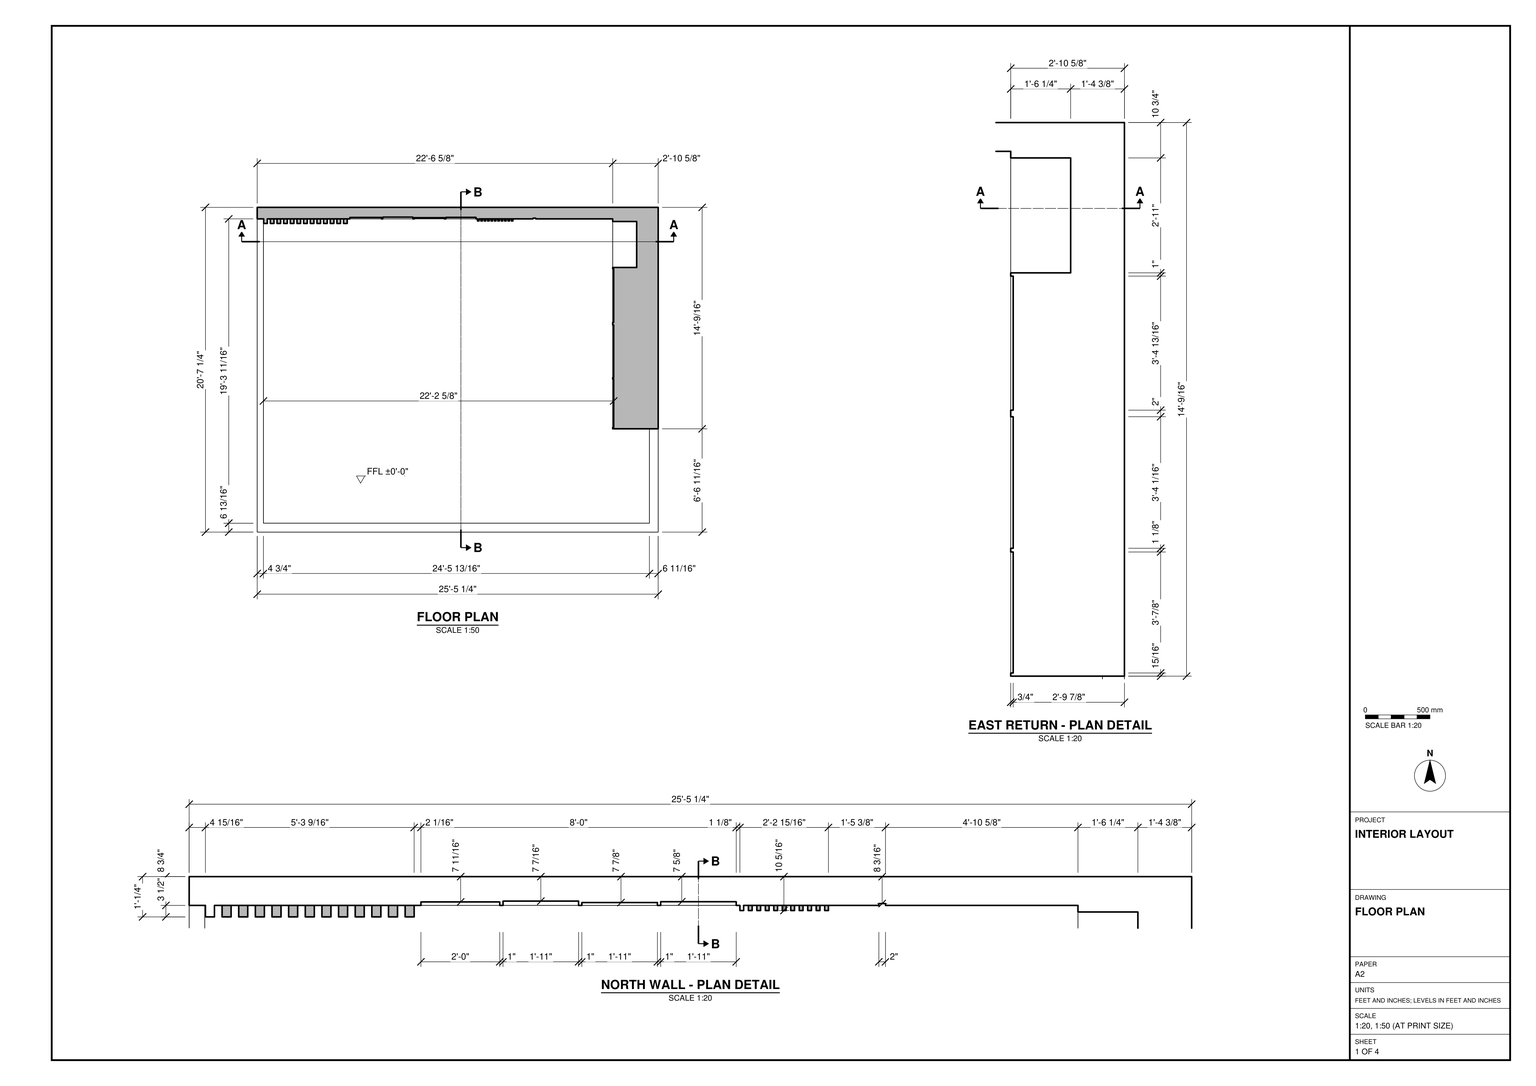
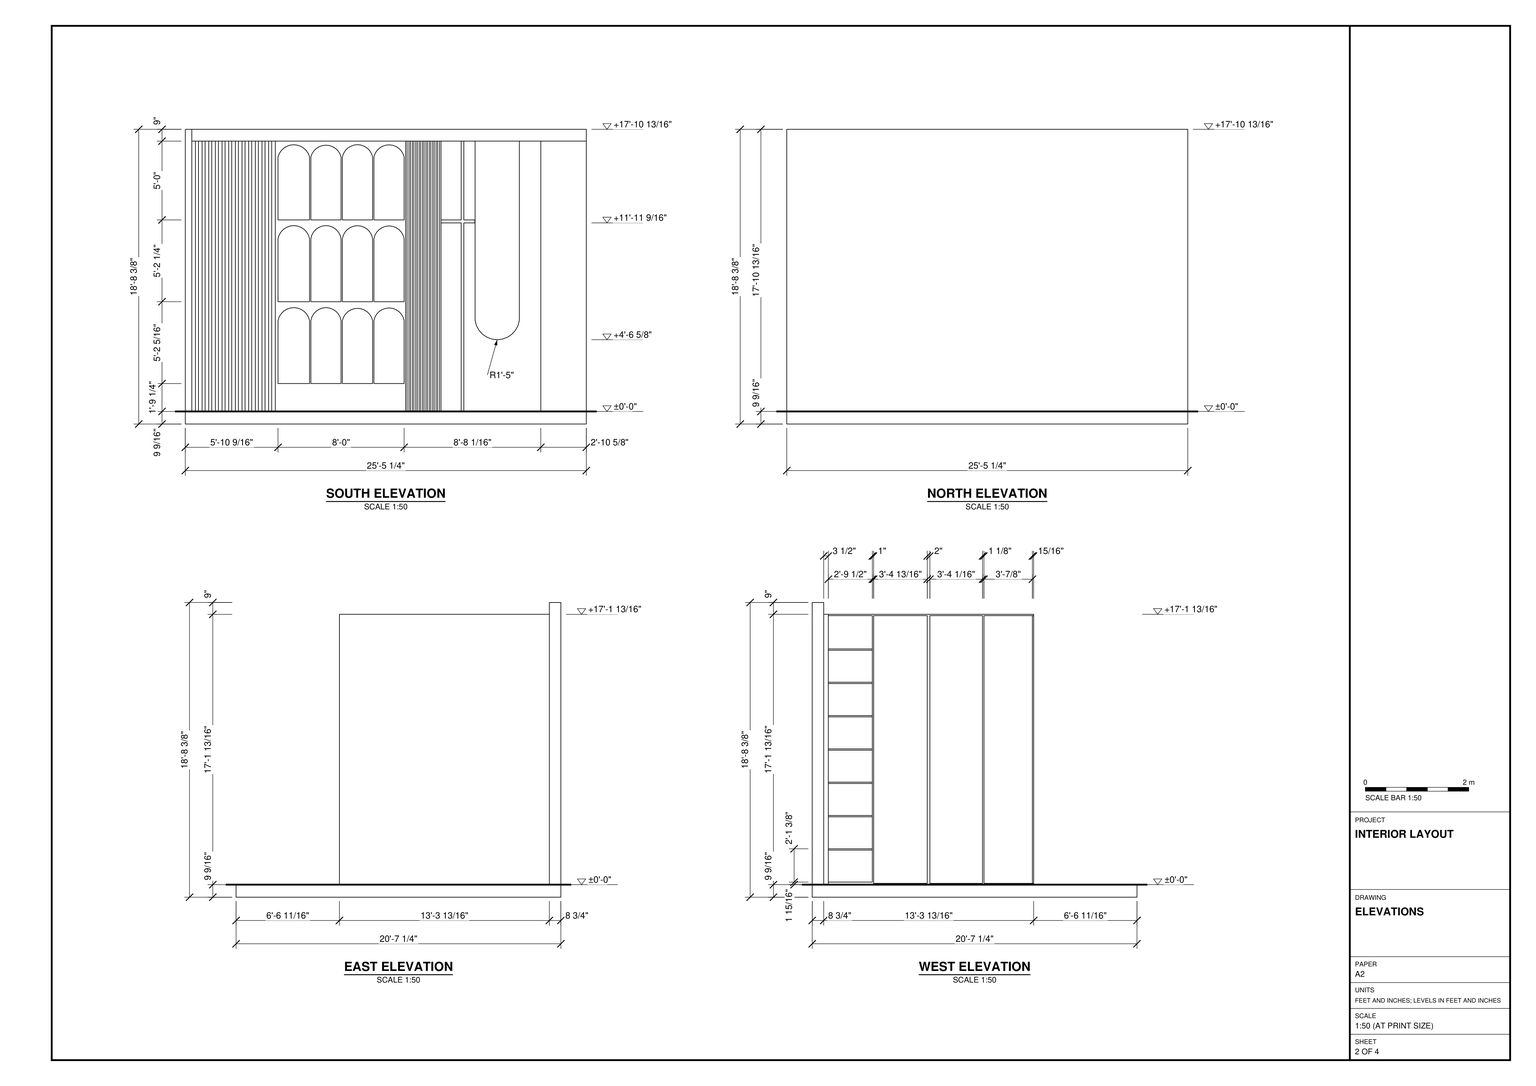
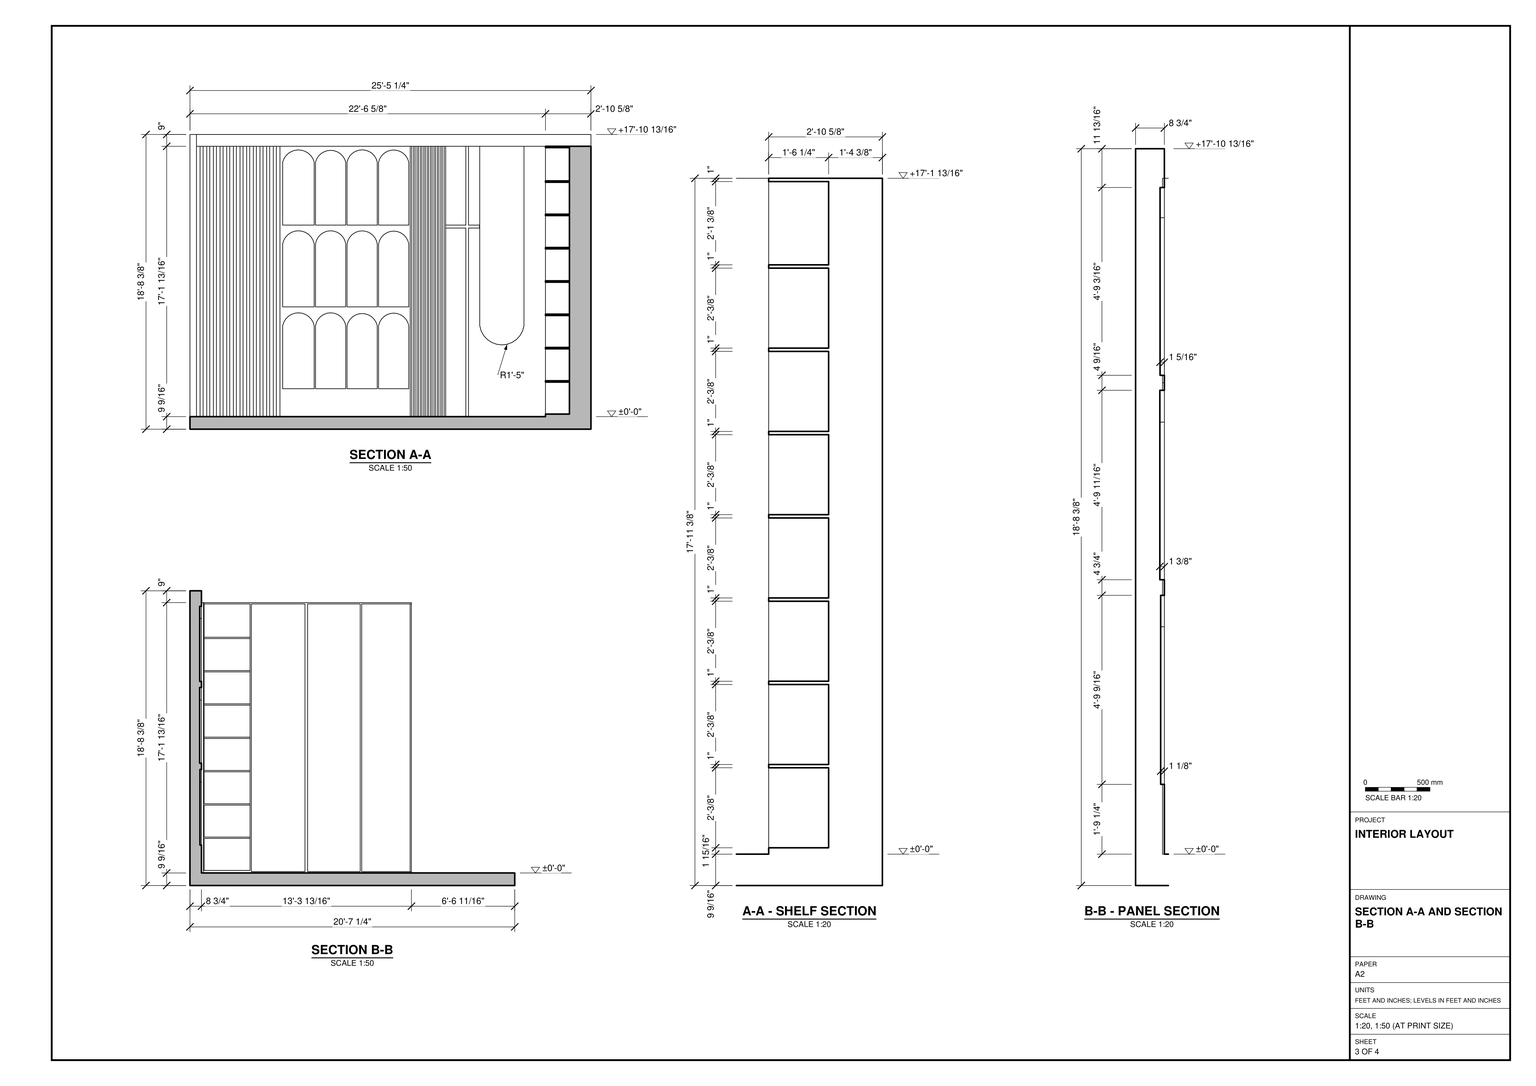
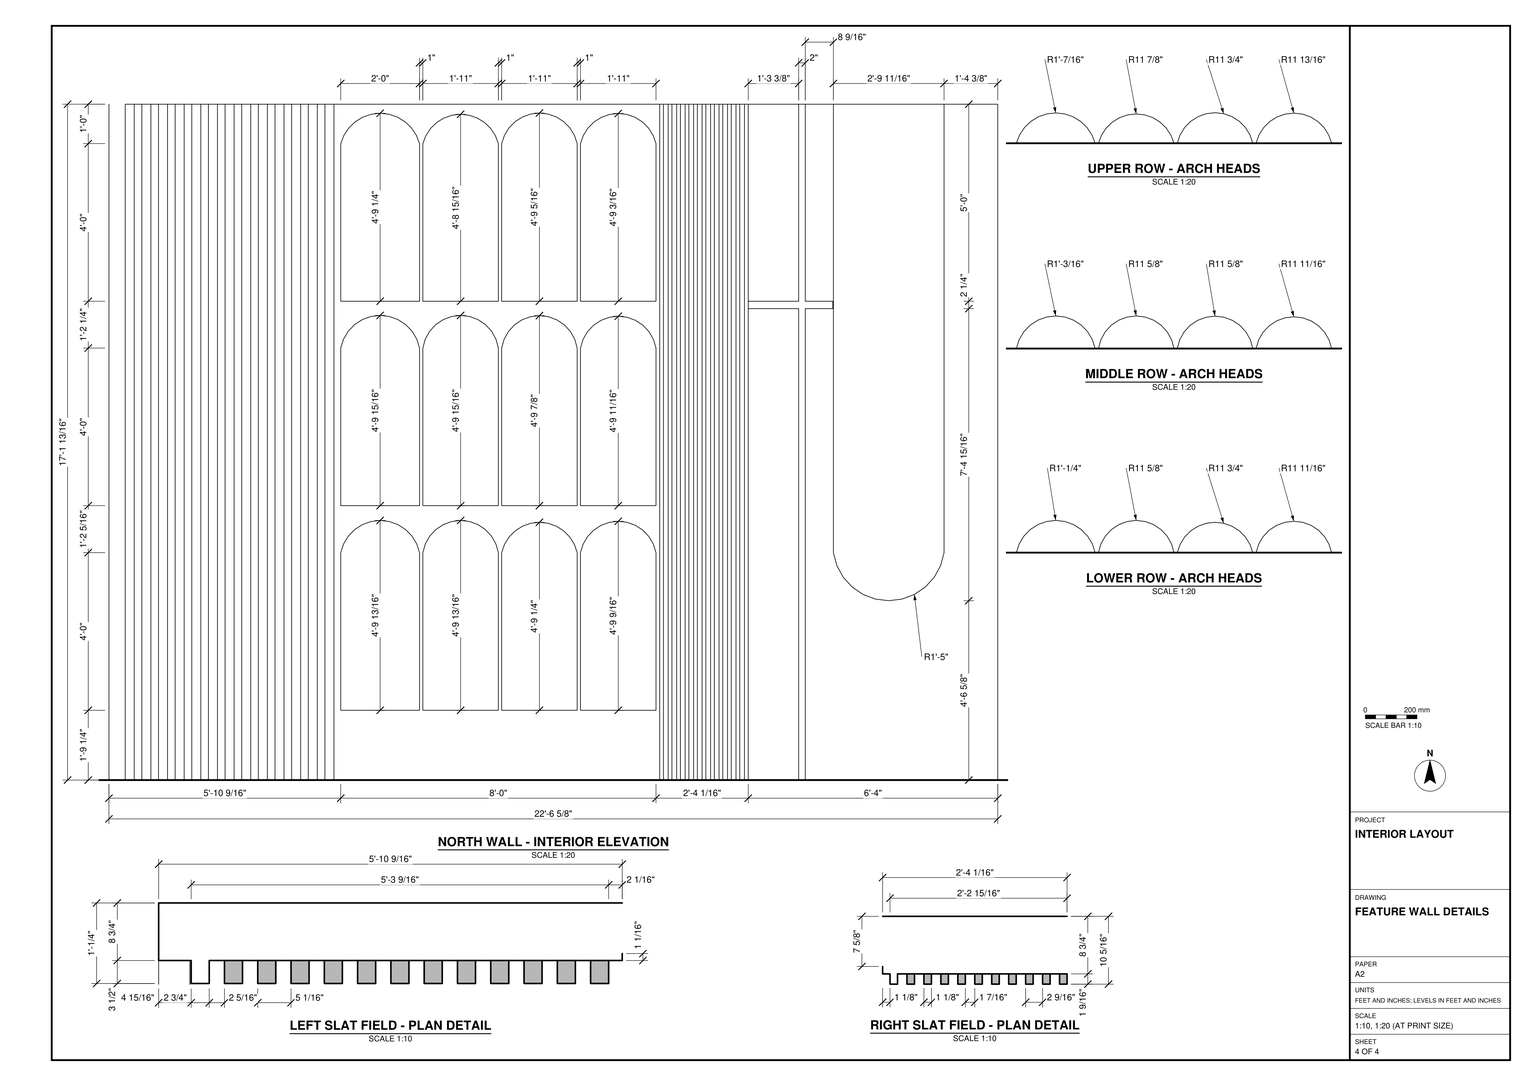
Use task_files/diagram_01.pdf to model the interior in SketchUp. Work in feet and inches. Set the finished floor at ±0'-0". The overall model measures 25'-5 1/4" east to west, 20'-7 1/4" north to south and 18'-8 3/8" from the underside of the slab to the top of the north wall.

Build the rectangular floor slab, the full-width north wall and the shorter east return. Use the plan details and sections for the wall thicknesses, panel offsets and shelf depths. On the room face of the north wall, place the field of round-headed panels between the broad and narrow bands of vertical slats. Follow the south elevation for the spacing of the arches, the clear strip above them and the tall panel with a rounded lower end toward the east corner. On the east return, place the open shelving nearest the north wall and the tall plain panels farther south. Leave the floor beyond the end of the return open as drawn.

Keep the slab, walls and individual joinery pieces in separate groups or components, and use components for repeated parts. Any decor or loose items shown may be represented by suitable library components. Save one SketchUp model as output_files/north_feature_wall_and_east_shelving_return.skp.

# SketchUp Ruby script. Lengths in inches.
U = 1.inch
M = Sketchup.active_model
def pt(a) = Geom::Point3d.new(a.map { |v| v * U })
def face(e, loops, mat)
  f = e.add_face(loops[0].map { |a| pt(a) })
  loops[1..].each { |l| e.add_face(l.map { |a| pt(a) }).erase! }
  f.material = f.back_material = mat if mat
  f
end
# faces: each face lists its corners as indices into pts; further lists are holes
def faces(e, pts, list, mat = nil) = list.each { |f| face(e, (f[0].is_a?(Array) ? f : [f]).map { |l| l.map { |i| pts[i] } }, mat) }
# xy, xz, yz: faces in a plane at the given z, y or x. An outline is a flat list of corners, or four numbers for a rectangle; further outlines are holes
def ring(l) = l.size == 4 ? [[l[0], l[1]], [l[2], l[1]], [l[2], l[3]], [l[0], l[3]]] : l.each_slice(2).to_a
def flat(e, list, mat, &to3) = list.each { |f| face(e, (f[0].is_a?(Array) ? f : [f]).map { |l| ring(l).map { |u, v| to3.(u, v) } }, mat) }
def xy(e, z, list, mat = nil) = flat(e, list, mat) { |x, y| [x, y, z] }
def xz(e, y, list, mat = nil) = flat(e, list, mat) { |x, z| [x, y, z] }
def yz(e, x, list, mat = nil) = flat(e, list, mat) { |y, z| [x, y, z] }
def lines(e, pts, list) = list.each { |a, b| e.add_line(pt(pts[a]), pt(pts[b])) }
# prism: a flat outline (further loops are holes) pulled along v
def prism(e, loops, v, mat = nil)
  f = face(e, loops, mat); d = Geom::Vector3d.new(v.map { |x| x * U })
  f.pushpull(f.normal.samedirection?(d) ? d.length : -d.length)
end
def box(e, o, s, mat = nil) = prism(e, [[o, [o[0] + s[0], o[1], o[2]], [o[0] + s[0], o[1] + s[1], o[2]], [o[0], o[1] + s[1], o[2]]]], [0, 0, s[2]], mat)
def at(x, y, z, deg = 0) = Geom::Transformation.translation(pt([x, y, z])) * Geom::Transformation.rotation(ORIGIN, Z_AXIS, deg.degrees)
def axes(o, x, y, z) = Geom::Transformation.new([*x, 0, *y, 0, *z, 0, *pt(o).to_a, 1])
def part(name) = M.definitions.add(name)
# library, detail: a bought-in or finely detailed component or shape, given as its bounding box
def library(name, o, s) = part(name).tap { |d| box(d.entities, o, s) }
def detail(e, o, s) = box(e.add_group.entities, o, s)
def put(e, d, t, mat = nil) = e.add_instance(d, t).tap { |i| i.material = mat if mat }
def group(e, t, mat = nil) = e.add_group.tap { |g| g.transformation = t; g.material = mat if mat }.entities
root = M.entities
xy(root,0,[[0,0,305.26,247.25]])
xy(root,9.5625,[[0,0,305.26,0,305.26,78.67,298.58,78.67,298.58,6.8125,4.75,6.8125,4.75,238.49,0,238.49],[4.75,6.8125,298.58,6.8125,298.58,78.67,270.64,78.67,270.64,238.49,212.04,238.49,212.04,239.05,210.01,239.05,210.01,238.49,194.66,238.49,194.66,236.92,193.51,236.92,193.51,238.49,192.08,238.49,192.08,236.92,190.93,236.92,190.93,238.49,189.5,238.49,189.5,236.92,188.35,236.92,188.35,238.49,186.91,238.49,186.91,236.92,185.77,236.92,185.77,238.49,184.33,238.49,184.33,236.92,183.19,236.92,183.19,238.49,181.75,238.49,181.75,236.92,180.61,236.92,180.61,238.49,179.17,238.49,179.17,236.92,178.03,236.92,178.03,238.49,176.59,238.49,176.59,236.92,175.45,236.92,175.45,238.49,174.01,238.49,174.01,236.92,172.86,236.92,172.86,238.49,171.43,238.49,171.43,236.92,170.28,236.92,170.28,238.49,168.85,238.49,168.85,236.92,167.7,236.92,167.7,238.49,68.51,238.49,68.51,234.99,65.76,234.99,65.76,238.49,63.44,238.49,63.44,234.99,60.7,234.99,60.7,238.49,58.375,238.49,58.375,234.99,55.63,234.99,55.63,238.49,53.31,238.49,53.31,234.99,50.5625,234.99,50.5625,238.49,48.24,238.49,48.24,234.99,45.49,234.99,45.49,238.49,43.17,238.49,43.17,234.99,40.43,234.99,40.43,238.49,38.1,238.49,38.1,234.99,35.36,234.99,35.36,238.49,33.04,238.49,33.04,234.99,30.29,234.99,30.29,238.49,27.97,238.49,27.97,234.99,25.22,234.99,25.22,238.49,22.9,238.49,22.9,234.99,20.16,234.99,20.16,238.49,17.83,238.49,17.83,234.99,15.09,234.99,15.09,238.49,12.77,238.49,12.77,234.99,10.02,234.99,10.02,238.49,7.7,238.49,7.7,234.99,4.95,234.99,4.95,238.49,4.75,238.49],[10.02,234.99,12.77,238.49],[15.09,234.99,17.83,238.49],[20.16,234.99,22.9,238.49],
  [25.22,234.99,27.97,238.49],[30.29,234.99,33.04,238.49],[35.36,234.99,38.1,238.49],[40.43,234.99,43.17,238.49],[45.49,234.99,48.24,238.49],
  [50.5625,234.99,53.31,238.49],[55.63,234.99,58.375,238.49],[60.7,234.99,63.44,238.49],[65.76,234.99,68.51,238.49],[170.28,236.92,171.43,238.49],
  [172.86,236.92,174.01,238.49],[175.45,236.92,176.59,238.49],[178.03,236.92,179.17,238.49],[180.61,236.92,181.75,238.49],[183.19,236.92,184.33,238.49],
  [185.77,236.92,186.91,238.49],[188.35,236.92,189.5,238.49],[190.93,236.92,192.08,238.49],[193.51,236.92,194.66,238.49]])
xy(root,10.5625,[[270.64,79.63,271.39,116.49],[270.64,117.61,271.39,157.67],[270.64,159.67,271.39,200.49]])
xy(root,11.5,[[270.64,201.49,288.89,236.49]])
xy(root,30.8125,[[70.58,238.49,94.58,239.55],[95.58,238.49,118.58,239.8],[119.58,238.49,142.58,239.36],[143.58,238.49,166.58,239.61]])
xy(root,35.87,[[270.64,201.49,288.89,236.49]])
xy(root,36.86,[[270.64,201.49,288.89,236.49]])
xy(root,61.22,[[270.64,201.49,288.89,236.49]])
xy(root,62.22,[[270.64,201.49,288.89,236.49]])
xy(root,86.58,[[270.64,201.49,288.89,236.49]])
xy(root,87.58,[[270.64,201.49,288.89,236.49]])
xy(root,93.125,[[70.58,238.49,94.58,239.36],[95.58,238.49,118.58,239.55],[119.58,238.49,142.58,239.86],[143.58,238.49,166.58,239.86]])
xy(root,111.9375,[[270.64,201.49,288.89,236.49]])
xy(root,112.9375,[[270.64,201.49,288.89,236.49]])
xy(root,137.3,[[270.64,201.49,288.89,236.49]])
xy(root,138.3,[[270.64,201.49,288.89,236.49]])
xy(root,153.125,[[194.66,238.49,210.01,239.05],[212.04,238.49,220.42,239.05]])
xy(root,155.375,[[70.58,238.49,94.58,239.61],[95.58,238.49,118.58,240.11],[119.58,238.49,142.58,239.8],[143.58,238.49,166.58,239.8],[194.66,238.49,210.01,239.05],
  [212.04,238.49,220.42,239.05]])
xy(root,162.66,[[270.64,201.49,288.89,236.49]])
xy(root,163.66,[[270.64,201.49,288.89,236.49]])
xy(root,188.02,[[270.64,201.49,288.89,236.49]])
xy(root,189.02,[[270.64,201.49,288.89,236.49]])
xy(root,214.375,[[270.64,79.63,271.39,116.49],[270.64,117.61,271.39,157.67],[270.64,159.67,271.39,200.49],[270.64,201.49,288.89,236.49]])
xy(root,215.375,[[270.64,78.67,305.26,238.49],[4.95,234.99,7.7,238.49],[10.02,234.99,12.77,238.49],[15.09,234.99,17.83,238.49],[20.16,234.99,22.9,238.49],
  [25.22,234.99,27.97,238.49],[30.29,234.99,33.04,238.49],[35.36,234.99,38.1,238.49],[40.43,234.99,43.17,238.49],[45.49,234.99,48.24,238.49],
  [50.5625,234.99,53.31,238.49],[55.63,234.99,58.375,238.49],[60.7,234.99,63.44,238.49],[65.76,234.99,68.51,238.49],[220.6,236.61,254.29,238.49],
  [167.7,236.92,168.85,238.49],[170.28,236.92,171.43,238.49],[172.86,236.92,174.01,238.49],[175.45,236.92,176.59,238.49],[178.03,236.92,179.17,238.49],
  [180.61,236.92,181.75,238.49],[183.19,236.92,184.33,238.49],[185.77,236.92,186.91,238.49],[188.35,236.92,189.5,238.49],[190.93,236.92,192.08,238.49],
  [193.51,236.92,194.66,238.49],[210.01,238.49,212.04,239.05]])
xy(root,224.375,[[0,238.49,305.26,247.25]])
xz(root,0,[[0,0,305.26,9.5625]])
xz(root,78.67,[[270.64,9.5625,305.26,215.375]])
xz(root,79.63,[[270.64,10.5625,271.39,214.375]])
xz(root,116.49,[[270.64,10.5625,271.39,214.375]])
xz(root,117.61,[[270.64,10.5625,271.39,214.375]])
xz(root,157.67,[[270.64,10.5625,271.39,214.375]])
xz(root,159.67,[[270.64,10.5625,271.39,214.375]])
xz(root,200.49,[[270.64,10.5625,271.39,214.375]])
xz(root,201.49,[[270.64,11.5,288.89,35.87],[270.64,35.87,288.89,36.86],[270.64,36.86,288.89,61.22],[270.64,61.22,288.89,62.22],[270.64,62.22,288.89,86.58],
  [270.64,86.58,288.89,87.58],[270.64,87.58,288.89,111.9375],[270.64,111.9375,288.89,112.9375],[270.64,112.9375,288.89,137.3],[270.64,137.3,288.89,138.3],
  [270.64,138.3,288.89,162.66],[270.64,162.66,288.89,163.66],[270.64,163.66,288.89,188.02],[270.64,188.02,288.89,189.02],[270.64,189.02,288.89,214.375]])
xz(root,234.99,[[4.95,9.5625,7.7,215.375],[10.02,9.5625,12.77,215.375],[15.09,9.5625,17.83,215.375],[20.16,9.5625,22.9,215.375],[25.22,9.5625,27.97,215.375],
  [30.29,9.5625,33.04,215.375],[35.36,9.5625,38.1,215.375],[40.43,9.5625,43.17,215.375],[45.49,9.5625,48.24,215.375],[50.5625,9.5625,53.31,215.375],
  [55.63,9.5625,58.375,215.375],[60.7,9.5625,63.44,215.375],[65.76,9.5625,68.51,215.375]])
xz(root,236.49,[[270.64,11.5,288.89,35.87],[270.64,36.86,288.89,61.22],[270.64,62.22,288.89,86.58],[270.64,87.58,288.89,111.9375],[270.64,112.9375,288.89,137.3],
  [270.64,138.3,288.89,162.66],[270.64,163.66,288.89,188.02],[270.64,189.02,288.89,214.375]])
xz(root,236.61,[[237.44,64.1875,241.46,64.67,245.25,66.08,248.59,68.35,251.3125,71.35,253.25,74.9,254.29,78.8125,254.29,215.375,220.6,215.375,220.6,78.8125,221.64,74.9,223.57,71.35,226.29,68.35,229.64,66.08,233.43,64.67]])
xz(root,236.92,[[167.7,9.5625,168.85,215.375],[170.28,9.5625,171.43,215.375],[172.86,9.5625,174.01,215.375],[175.45,9.5625,176.59,215.375],[178.03,9.5625,179.17,215.375],
  [180.61,9.5625,181.75,215.375],[183.19,9.5625,184.33,215.375],[185.77,9.5625,186.91,215.375],[188.35,9.5625,189.5,215.375],[190.93,9.5625,192.08,215.375],
  [193.51,9.5625,194.66,215.375]])
xz(root,238.49,[[0,9.5625,4.95,224.375],[7.7,9.5625,10.02,215.375],[10.02,9.5625,12.77,215.375],[12.77,9.5625,15.09,215.375],[15.09,9.5625,17.83,215.375],
  [17.83,9.5625,20.16,215.375],[20.16,9.5625,22.9,215.375],[22.9,9.5625,25.22,215.375],[25.22,9.5625,27.97,215.375],[27.97,9.5625,30.29,215.375],
  [30.29,9.5625,33.04,215.375],[33.04,9.5625,35.36,215.375],[35.36,9.5625,38.1,215.375],[38.1,9.5625,40.43,215.375],[40.43,9.5625,43.17,215.375],
  [43.17,9.5625,45.49,215.375],[45.49,9.5625,48.24,215.375],[48.24,9.5625,50.5625,215.375],[50.5625,9.5625,53.31,215.375],[53.31,9.5625,55.63,215.375],
  [55.63,9.5625,58.375,215.375],[58.375,9.5625,60.7,215.375],[60.7,9.5625,63.44,215.375],[63.44,9.5625,65.76,215.375],[65.76,9.5625,68.51,215.375],
  [[68.51,9.5625,167.7,215.375],[70.58,93.125,70.58,141.125,71.41,143.81,72.84,146.23,74.79,148.26,77.14,149.79,79.79,150.74,82.58,151.0625,85.37,150.74,88.01,149.79,90.37,148.26,92.3125,146.23,93.74,143.81,94.58,141.125,94.58,93.125],[70.58,30.8125,70.58,78.8125,71.44,81.47,72.88,83.86,74.83,85.86,77.17,87.37,79.8,88.31,82.58,88.625,85.35,88.31,87.98,87.37,90.33,85.86,92.27,83.86,93.71,81.47,94.58,78.8125,94.58,30.8125],[70.58,155.375,70.58,203.375,71.55,205.91,73.05,208.16,75,210.04,77.32,211.45,79.88,212.33,82.58,212.625,85.27,212.33,87.84,211.45,90.15,210.04,92.11,208.16,93.6,205.91,94.58,203.375,94.58,155.375],[95.58,93.125,95.58,141.125,96.3,143.78,97.62,146.2,99.48,148.23,101.76,149.78,104.34,150.74,107.08,151.0625,109.8125,150.74,112.39,149.78,114.68,148.23,116.53,146.2,117.86,143.78,118.58,141.125,118.58,93.125],[119.58,93.125,119.58,141.125,120.31,143.77,121.64,146.17,123.5,148.19,125.78,149.72,128.35,150.68,131.08,151,133.8,150.68,136.375,149.72,138.66,148.19,140.51,146.17,141.84,143.77,142.58,141.125,142.58,93.125],[95.58,30.8125,95.58,78.8125,96.32,81.44,97.66,83.83,99.52,85.84,101.79,87.36,104.36,88.3,107.08,88.625,109.79,88.3,112.36,87.36,114.64,85.84,116.49,83.83,117.83,81.44,118.58,78.8125,118.58,30.8125],[143.58,93.125,143.58,141.125,144.35,143.73,145.7,146.09,147.56,148.07,149.83,149.5625,152.38,150.5,155.08,150.8125,157.78,150.5,160.33,149.5625,162.6,148.07,164.46,146.09,165.81,143.73,166.58,141.125,166.58,93.125],[143.58,30.8125,143.58,78.8125,144.37,81.39,145.74,83.72,147.6,85.67,149.86,87.15,152.4,88.0625,155.08,88.375,157.76,88.0625,160.3,87.15,162.56,85.67,164.42,83.72,165.78,81.39,166.58,78.8125,166.58,30.8125],[119.58,155.375,119.58,203.375,120.42,205.9,121.8125,208.17,123.68,210.07,125.92,211.5,128.43,212.39,131.08,212.6875,133.72,212.39,136.23,211.5,138.48,210.07,140.34,208.17,141.73,205.9,142.58,203.375,142.58,155.375],[119.58,30.8125,119.58,78.8125,120.43,81.32,121.83,83.58,123.7,85.46,125.9375,86.88,128.44,87.76,131.08,88.0625,133.71,87.76,136.22,86.88,138.46,85.46,140.32,83.58,141.72,81.32,142.58,78.8125,142.58,30.8125],[143.58,155.375,143.58,203.375,144.45,205.87,145.85,208.11,147.72,209.98,149.95,211.39,152.45,212.27,155.08,212.5625,157.7,212.27,160.2,211.39,162.4375,209.98,164.3,208.11,165.71,205.87,166.58,203.375,166.58,155.375],[95.58,155.375,95.58,203.375,96.49,205.82,97.92,208,99.79,209.82,102.02,211.18,104.48,212.03,107.08,212.3125,109.67,212.03,112.14,211.18,114.36,209.82,116.23,208,117.66,205.82,118.58,203.375,118.58,155.375]],[168.85,9.5625,170.28,215.375],[170.28,9.5625,171.43,215.375],[171.43,9.5625,172.86,215.375],[172.86,9.5625,174.01,215.375],
  [174.01,9.5625,175.45,215.375],[175.45,9.5625,176.59,215.375],[176.59,9.5625,178.03,215.375],[178.03,9.5625,179.17,215.375],[179.17,9.5625,180.61,215.375],
  [180.61,9.5625,181.75,215.375],[181.75,9.5625,183.19,215.375],[183.19,9.5625,184.33,215.375],[184.33,9.5625,185.77,215.375],[185.77,9.5625,186.91,215.375],
  [186.91,9.5625,188.35,215.375],[188.35,9.5625,189.5,215.375],[189.5,9.5625,190.93,215.375],[190.93,9.5625,192.08,215.375],[192.08,9.5625,193.51,215.375],
  [193.51,9.5625,194.66,215.375],[194.66,9.5625,210.01,153.125],[212.04,9.5625,270.64,9.5625,270.64,215.375,254.29,215.375,254.29,78.8125,253.25,74.9,251.3125,71.35,248.59,68.35,245.25,66.08,241.46,64.67,237.44,64.1875,233.43,64.67,229.64,66.08,226.29,68.35,223.57,71.35,221.64,74.9,220.6,78.8125,220.6,215.375,212.04,215.375,212.04,155.375,220.42,155.375,220.42,153.125,212.04,153.125],[194.66,155.375,210.01,215.375],[4.95,215.375,305.26,224.375]])
xz(root,239.05,[[210.01,9.5625,212.04,9.5625,212.04,153.125,220.42,153.125,220.42,155.375,212.04,155.375,212.04,215.375,210.01,215.375,210.01,155.375,194.66,155.375,194.66,153.125,210.01,153.125]])
xz(root,239.36,[[119.58,30.8125,142.58,30.8125,142.58,78.8125,141.72,81.32,140.32,83.58,138.46,85.46,136.22,86.88,133.71,87.76,131.08,88.0625,128.44,87.76,125.9375,86.88,123.7,85.46,121.83,83.58,120.43,81.32,119.58,78.8125],[70.58,93.125,94.58,93.125,94.58,141.125,93.74,143.81,92.3125,146.23,90.37,148.26,88.01,149.79,85.37,150.74,82.58,151.0625,79.79,150.74,77.14,149.79,74.79,148.26,72.84,146.23,71.41,143.81,70.58,141.125]])
xz(root,239.55,[[70.58,30.8125,94.58,30.8125,94.58,78.8125,93.71,81.47,92.27,83.86,90.33,85.86,87.98,87.37,85.35,88.31,82.58,88.625,79.8,88.31,77.17,87.37,74.83,85.86,72.88,83.86,71.44,81.47,70.58,78.8125],[95.58,93.125,118.58,93.125,118.58,141.125,117.86,143.78,116.53,146.2,114.68,148.23,112.39,149.78,109.8125,150.74,107.08,151.0625,104.34,150.74,101.76,149.78,99.48,148.23,97.62,146.2,96.3,143.78,95.58,141.125]])
xz(root,239.61,[[143.58,30.8125,166.58,30.8125,166.58,78.8125,165.78,81.39,164.42,83.72,162.56,85.67,160.3,87.15,157.76,88.0625,155.08,88.375,152.4,88.0625,149.86,87.15,147.6,85.67,145.74,83.72,144.37,81.39,143.58,78.8125],[70.58,155.375,94.58,155.375,94.58,203.375,93.6,205.91,92.11,208.16,90.15,210.04,87.84,211.45,85.27,212.33,82.58,212.625,79.88,212.33,77.32,211.45,75,210.04,73.05,208.16,71.55,205.91,70.58,203.375]])
xz(root,239.8,[[95.58,30.8125,118.58,30.8125,118.58,78.8125,117.83,81.44,116.49,83.83,114.64,85.84,112.36,87.36,109.79,88.3,107.08,88.625,104.36,88.3,101.79,87.36,99.52,85.84,97.66,83.83,96.32,81.44,95.58,78.8125],[119.58,155.375,142.58,155.375,142.58,203.375,141.73,205.9,140.34,208.17,138.48,210.07,136.23,211.5,133.72,212.39,131.08,212.6875,128.43,212.39,125.92,211.5,123.68,210.07,121.8125,208.17,120.42,205.9,119.58,203.375],[143.58,155.375,166.58,155.375,166.58,203.375,165.71,205.87,164.3,208.11,162.4375,209.98,160.2,211.39,157.7,212.27,155.08,212.5625,152.45,212.27,149.95,211.39,147.72,209.98,145.85,208.11,144.45,205.87,143.58,203.375]])
xz(root,239.86,[[119.58,93.125,142.58,93.125,142.58,141.125,141.84,143.77,140.51,146.17,138.66,148.19,136.375,149.72,133.8,150.68,131.08,151,128.35,150.68,125.78,149.72,123.5,148.19,121.64,146.17,120.31,143.77,119.58,141.125],[143.58,93.125,166.58,93.125,166.58,141.125,165.81,143.73,164.46,146.09,162.6,148.07,160.33,149.5625,157.78,150.5,155.08,150.8125,152.38,150.5,149.83,149.5625,147.56,148.07,145.7,146.09,144.35,143.73,143.58,141.125]])
xz(root,240.11,[[95.58,155.375,118.58,155.375,118.58,203.375,117.66,205.82,116.23,208,114.36,209.82,112.14,211.18,109.67,212.03,107.08,212.3125,104.48,212.03,102.02,211.18,99.79,209.82,97.92,208,96.49,205.82,95.58,203.375]])
xz(root,247.25,[[0,0,305.26,224.375]])
yz(root,0,[[0,0,0,9.5625,238.49,9.5625,238.49,224.375,247.25,224.375,247.25,0]])
yz(root,4.95,[[234.99,9.5625,238.49,215.375]])
yz(root,7.7,[[234.99,9.5625,238.49,215.375]])
yz(root,10.02,[[234.99,9.5625,238.49,215.375]])
yz(root,12.77,[[234.99,9.5625,238.49,215.375]])
yz(root,15.09,[[234.99,9.5625,238.49,215.375]])
yz(root,17.83,[[234.99,9.5625,238.49,215.375]])
yz(root,20.16,[[234.99,9.5625,238.49,215.375]])
yz(root,22.9,[[234.99,9.5625,238.49,215.375]])
yz(root,25.22,[[234.99,9.5625,238.49,215.375]])
yz(root,27.97,[[234.99,9.5625,238.49,215.375]])
yz(root,30.29,[[234.99,9.5625,238.49,215.375]])
yz(root,33.04,[[234.99,9.5625,238.49,215.375]])
yz(root,35.36,[[234.99,9.5625,238.49,215.375]])
yz(root,38.1,[[234.99,9.5625,238.49,215.375]])
yz(root,40.43,[[234.99,9.5625,238.49,215.375]])
yz(root,43.17,[[234.99,9.5625,238.49,215.375]])
yz(root,45.49,[[234.99,9.5625,238.49,215.375]])
yz(root,48.24,[[234.99,9.5625,238.49,215.375]])
yz(root,50.5625,[[234.99,9.5625,238.49,215.375]])
yz(root,53.31,[[234.99,9.5625,238.49,215.375]])
yz(root,55.63,[[234.99,9.5625,238.49,215.375]])
yz(root,58.375,[[234.99,9.5625,238.49,215.375]])
yz(root,60.7,[[234.99,9.5625,238.49,215.375]])
yz(root,63.44,[[234.99,9.5625,238.49,215.375]])
yz(root,65.76,[[234.99,9.5625,238.49,215.375]])
yz(root,68.51,[[234.99,9.5625,238.49,215.375]])
yz(root,70.58,[[238.49,30.8125,239.55,78.8125],[238.49,93.125,239.36,141.125],[238.49,155.375,239.61,203.375]])
yz(root,94.58,[[238.49,30.8125,239.55,78.8125],[238.49,93.125,239.36,141.125],[238.49,155.375,239.61,203.375]])
yz(root,95.58,[[238.49,30.8125,239.8,78.8125],[238.49,93.125,239.55,141.125],[238.49,155.375,240.11,203.375]])
yz(root,118.58,[[238.49,30.8125,239.8,78.8125],[238.49,93.125,239.55,141.125],[238.49,155.375,240.11,203.375]])
yz(root,119.58,[[238.49,30.8125,239.36,78.8125],[238.49,93.125,239.86,141.125],[238.49,155.375,239.8,203.375]])
yz(root,142.58,[[238.49,30.8125,239.36,78.8125],[238.49,93.125,239.86,141.125],[238.49,155.375,239.8,203.375]])
yz(root,143.58,[[238.49,30.8125,239.61,78.8125],[238.49,93.125,239.86,141.125],[238.49,155.375,239.8,203.375]])
yz(root,166.58,[[238.49,30.8125,239.61,78.8125],[238.49,93.125,239.86,141.125],[238.49,155.375,239.8,203.375]])
yz(root,167.7,[[236.92,9.5625,238.49,215.375]])
yz(root,168.85,[[236.92,9.5625,238.49,215.375]])
yz(root,170.28,[[236.92,9.5625,238.49,215.375]])
yz(root,171.43,[[236.92,9.5625,238.49,215.375]])
yz(root,172.86,[[236.92,9.5625,238.49,215.375]])
yz(root,174.01,[[236.92,9.5625,238.49,215.375]])
yz(root,175.45,[[236.92,9.5625,238.49,215.375]])
yz(root,176.59,[[236.92,9.5625,238.49,215.375]])
yz(root,178.03,[[236.92,9.5625,238.49,215.375]])
yz(root,179.17,[[236.92,9.5625,238.49,215.375]])
yz(root,180.61,[[236.92,9.5625,238.49,215.375]])
yz(root,181.75,[[236.92,9.5625,238.49,215.375]])
yz(root,183.19,[[236.92,9.5625,238.49,215.375]])
yz(root,184.33,[[236.92,9.5625,238.49,215.375]])
yz(root,185.77,[[236.92,9.5625,238.49,215.375]])
yz(root,186.91,[[236.92,9.5625,238.49,215.375]])
yz(root,188.35,[[236.92,9.5625,238.49,215.375]])
yz(root,189.5,[[236.92,9.5625,238.49,215.375]])
yz(root,190.93,[[236.92,9.5625,238.49,215.375]])
yz(root,192.08,[[236.92,9.5625,238.49,215.375]])
yz(root,193.51,[[236.92,9.5625,238.49,215.375]])
yz(root,194.66,[[236.92,9.5625,238.49,215.375],[238.49,153.125,239.05,155.375]])
yz(root,210.01,[[238.49,9.5625,239.05,153.125],[238.49,155.375,239.05,215.375]])
yz(root,212.04,[[238.49,9.5625,239.05,153.125],[238.49,155.375,239.05,215.375]])
yz(root,220.42,[[238.49,153.125,239.05,155.375]])
yz(root,220.6,[[236.61,78.8125,238.49,215.375]])
yz(root,254.29,[[236.61,78.8125,238.49,215.375]])
yz(root,270.64,[[[78.67,9.5625,78.67,10.5625,116.49,10.5625,116.49,214.375,78.67,214.375,78.67,215.375,238.49,215.375,238.49,9.5625],[159.67,10.5625,200.49,214.375],[117.61,10.5625,157.67,214.375],[201.49,189.02,236.49,214.375],[201.49,11.5,236.49,35.87],[201.49,163.66,236.49,188.02],[201.49,138.3,236.49,162.66],[201.49,112.9375,236.49,137.3],[201.49,87.58,236.49,111.9375],[201.49,62.22,236.49,86.58],[201.49,36.86,236.49,61.22]],[78.67,10.5625,79.63,214.375]])
yz(root,271.39,[[79.63,10.5625,116.49,214.375],[117.61,10.5625,157.67,214.375],[159.67,10.5625,200.49,214.375]])
yz(root,288.89,[[201.49,11.5,236.49,35.87],[201.49,36.86,236.49,61.22],[201.49,62.22,236.49,86.58],[201.49,87.58,236.49,111.9375],[201.49,112.9375,236.49,137.3],
  [201.49,138.3,236.49,162.66],[201.49,163.66,236.49,188.02],[201.49,189.02,236.49,214.375]])
yz(root,305.26,[[0,0,247.25,0,247.25,224.375,238.49,224.375,238.49,9.5625,0,9.5625],[78.67,9.5625,238.49,215.375]])
p = [[233.43,238.49,64.67],[237.44,238.49,64.1875],[237.44,236.61,64.1875],[233.43,236.61,64.67],[241.46,238.49,64.67],[241.46,236.61,64.67],
  [229.64,238.49,66.08],[229.64,236.61,66.08],[245.25,238.49,66.08],[245.25,236.61,66.08],[226.29,238.49,68.35],[226.29,236.61,68.35],
  [248.59,238.49,68.35],[248.59,236.61,68.35],[223.57,238.49,71.35],[223.57,236.61,71.35],[251.3125,238.49,71.35],[251.3125,236.61,71.35],
  [221.64,238.49,74.9],[221.64,236.61,74.9],[253.25,238.49,74.9],[253.25,236.61,74.9],[220.6,238.49,78.8125],[220.6,236.61,78.8125],
  [254.29,238.49,78.8125],[254.29,236.61,78.8125],[71.44,238.49,81.47],[70.58,238.49,78.8125],[70.58,239.55,78.8125],[71.44,239.55,81.47],
  [94.58,238.49,78.8125],[93.71,238.49,81.47],[93.71,239.55,81.47],[94.58,239.55,78.8125],[96.32,238.49,81.44],[95.58,238.49,78.8125],
  [95.58,239.8,78.8125],[96.32,239.8,81.44],[118.58,238.49,78.8125],[117.83,238.49,81.44],[117.83,239.8,81.44],[118.58,239.8,78.8125],
  [120.43,238.49,81.32],[119.58,238.49,78.8125],[119.58,239.36,78.8125],[120.43,239.36,81.32],[142.58,238.49,78.8125],[141.72,238.49,81.32],
  [141.72,239.36,81.32],[142.58,239.36,78.8125],[144.37,238.49,81.39],[143.58,238.49,78.8125],[143.58,239.61,78.8125],[144.37,239.61,81.39],
  [166.58,238.49,78.8125],[165.78,238.49,81.39],[165.78,239.61,81.39],[166.58,239.61,78.8125],[121.83,238.49,83.58],[121.83,239.36,83.58],
  [140.32,238.49,83.58],[140.32,239.36,83.58],[97.66,238.49,83.83],[97.66,239.8,83.83],[116.49,238.49,83.83],[116.49,239.8,83.83],
  [145.74,238.49,83.72],[145.74,239.61,83.72],[164.42,238.49,83.72],[164.42,239.61,83.72],[72.88,238.49,83.86],[72.88,239.55,83.86],
  [92.27,238.49,83.86],[92.27,239.55,83.86],[123.7,238.49,85.46],[123.7,239.36,85.46],[138.46,238.49,85.46],[138.46,239.36,85.46],
  [147.6,238.49,85.67],[147.6,239.61,85.67],[162.56,238.49,85.67],[162.56,239.61,85.67],[99.52,238.49,85.84],[99.52,239.8,85.84],
  [114.64,238.49,85.84],[114.64,239.8,85.84],[74.83,238.49,85.86],[74.83,239.55,85.86],[90.33,238.49,85.86],[90.33,239.55,85.86],
  [125.9375,238.49,86.88],[125.9375,239.36,86.88],[136.22,238.49,86.88],[136.22,239.36,86.88],[149.86,238.49,87.15],[149.86,239.61,87.15],
  [160.3,238.49,87.15],[160.3,239.61,87.15],[101.79,238.49,87.36],[101.79,239.8,87.36],[112.36,238.49,87.36],[112.36,239.8,87.36],
  [77.17,238.49,87.37],[77.17,239.55,87.37],[87.98,238.49,87.37],[87.98,239.55,87.37],[128.44,238.49,87.76],[128.44,239.36,87.76],
  [133.71,238.49,87.76],[133.71,239.36,87.76],[152.4,238.49,88.0625],[152.4,239.61,88.0625],[157.76,238.49,88.0625],[157.76,239.61,88.0625],
  [79.8,238.49,88.31],[79.8,239.55,88.31],[85.35,238.49,88.31],[85.35,239.55,88.31],[104.36,238.49,88.3],[104.36,239.8,88.3],
  [109.79,238.49,88.3],[109.79,239.8,88.3],[131.08,238.49,88.0625],[131.08,239.36,88.0625],[155.08,238.49,88.375],[155.08,239.61,88.375],
  [82.58,238.49,88.625],[82.58,239.55,88.625],[107.08,238.49,88.625],[107.08,239.8,88.625],[71.41,238.49,143.81],[70.58,238.49,141.125],
  [70.58,239.36,141.125],[71.41,239.36,143.81],[94.58,238.49,141.125],[93.74,238.49,143.81],[93.74,239.36,143.81],[94.58,239.36,141.125],
  [96.3,238.49,143.78],[95.58,238.49,141.125],[95.58,239.55,141.125],[96.3,239.55,143.78],[118.58,238.49,141.125],[117.86,238.49,143.78],
  [117.86,239.55,143.78],[118.58,239.55,141.125],[120.31,238.49,143.77],[119.58,238.49,141.125],[119.58,239.86,141.125],[120.31,239.86,143.77],
  [142.58,238.49,141.125],[141.84,238.49,143.77],[141.84,239.86,143.77],[142.58,239.86,141.125],[144.35,238.49,143.73],[143.58,238.49,141.125],
  [143.58,239.86,141.125],[144.35,239.86,143.73],[166.58,238.49,141.125],[165.81,238.49,143.73],[165.81,239.86,143.73],[166.58,239.86,141.125],
  [145.7,238.49,146.09],[145.7,239.86,146.09],[164.46,238.49,146.09],[164.46,239.86,146.09],[72.84,238.49,146.23],[72.84,239.36,146.23],
  [92.3125,238.49,146.23],[92.3125,239.36,146.23],[97.62,238.49,146.2],[97.62,239.55,146.2],[116.53,238.49,146.2],[116.53,239.55,146.2],
  [121.64,238.49,146.17],[121.64,239.86,146.17],[140.51,238.49,146.17],[140.51,239.86,146.17],[147.56,238.49,148.07],[147.56,239.86,148.07],
  [162.6,238.49,148.07],[162.6,239.86,148.07],[74.79,238.49,148.26],[74.79,239.36,148.26],[90.37,238.49,148.26],[90.37,239.36,148.26],
  [99.48,238.49,148.23],[99.48,239.55,148.23],[114.68,238.49,148.23],[114.68,239.55,148.23],[123.5,238.49,148.19],[123.5,239.86,148.19],
  [138.66,238.49,148.19],[138.66,239.86,148.19],[149.83,238.49,149.5625],[149.83,239.86,149.5625],[160.33,238.49,149.5625],[160.33,239.86,149.5625],
  [101.76,238.49,149.78],[101.76,239.55,149.78],[112.39,238.49,149.78],[112.39,239.55,149.78],[125.78,238.49,149.72],[125.78,239.86,149.72],
  [136.375,238.49,149.72],[136.375,239.86,149.72],[77.14,238.49,149.79],[77.14,239.36,149.79],[88.01,238.49,149.79],[88.01,239.36,149.79],
  [152.38,238.49,150.5],[152.38,239.86,150.5],[157.78,238.49,150.5],[157.78,239.86,150.5],[128.35,238.49,150.68],[128.35,239.86,150.68],
  [133.8,238.49,150.68],[133.8,239.86,150.68],[79.79,238.49,150.74],[79.79,239.36,150.74],[85.37,238.49,150.74],[85.37,239.36,150.74],
  [104.34,238.49,150.74],[104.34,239.55,150.74],[109.8125,238.49,150.74],[109.8125,239.55,150.74],[155.08,238.49,150.8125],[155.08,239.86,150.8125],
  [82.58,238.49,151.0625],[82.58,239.36,151.0625],[107.08,238.49,151.0625],[107.08,239.55,151.0625],[131.08,238.49,151],[131.08,239.86,151],
  [71.55,238.49,205.91],[70.58,238.49,203.375],[70.58,239.61,203.375],[71.55,239.61,205.91],[94.58,238.49,203.375],[93.6,238.49,205.91],
  [93.6,239.61,205.91],[94.58,239.61,203.375],[96.49,238.49,205.82],[95.58,238.49,203.375],[95.58,240.11,203.375],[96.49,240.11,205.82],
  [118.58,238.49,203.375],[117.66,238.49,205.82],[117.66,240.11,205.82],[118.58,240.11,203.375],[120.42,238.49,205.9],[119.58,238.49,203.375],
  [119.58,239.8,203.375],[120.42,239.8,205.9],[142.58,238.49,203.375],[141.73,238.49,205.9],[141.73,239.8,205.9],[142.58,239.8,203.375],
  [144.45,238.49,205.87],[143.58,238.49,203.375],[143.58,239.8,203.375],[144.45,239.8,205.87],[166.58,238.49,203.375],[165.71,238.49,205.87],
  [165.71,239.8,205.87],[166.58,239.8,203.375],[97.92,238.49,208],[97.92,240.11,208],[116.23,238.49,208],[116.23,240.11,208],
  [73.05,238.49,208.16],[73.05,239.61,208.16],[92.11,238.49,208.16],[92.11,239.61,208.16],[121.8125,238.49,208.17],[121.8125,239.8,208.17],
  [140.34,238.49,208.17],[140.34,239.8,208.17],[145.85,238.49,208.11],[145.85,239.8,208.11],[164.3,238.49,208.11],[164.3,239.8,208.11],
  [99.79,238.49,209.82],[99.79,240.11,209.82],[114.36,238.49,209.82],[114.36,240.11,209.82],[147.72,238.49,209.98],[147.72,239.8,209.98],
  [162.4375,238.49,209.98],[162.4375,239.8,209.98],[75,238.49,210.04],[75,239.61,210.04],[90.15,238.49,210.04],[90.15,239.61,210.04],
  [123.68,238.49,210.07],[123.68,239.8,210.07],[138.48,238.49,210.07],[138.48,239.8,210.07],[102.02,238.49,211.18],[102.02,240.11,211.18],
  [112.14,238.49,211.18],[112.14,240.11,211.18],[77.32,238.49,211.45],[77.32,239.61,211.45],[87.84,238.49,211.45],[87.84,239.61,211.45],
  [149.95,238.49,211.39],[149.95,239.8,211.39],[160.2,238.49,211.39],[160.2,239.8,211.39],[125.92,238.49,211.5],[125.92,239.8,211.5],
  [136.23,238.49,211.5],[136.23,239.8,211.5],[104.48,238.49,212.03],[104.48,240.11,212.03],[109.67,238.49,212.03],[109.67,240.11,212.03],
  [152.45,238.49,212.27],[152.45,239.8,212.27],[157.7,238.49,212.27],[157.7,239.8,212.27],[79.88,238.49,212.33],[79.88,239.61,212.33],
  [85.27,238.49,212.33],[85.27,239.61,212.33],[128.43,238.49,212.39],[128.43,239.8,212.39],[133.72,238.49,212.39],[133.72,239.8,212.39],
  [107.08,238.49,212.3125],[107.08,240.11,212.3125],[82.58,238.49,212.625],[82.58,239.61,212.625],[155.08,238.49,212.5625],[155.08,239.8,212.5625],
  [131.08,238.49,212.6875],[131.08,239.8,212.6875]]
faces(root,p,[[0,1,2,3],[1,4,5,2],[6,0,3,7],[4,8,9,5],[10,6,7,11],[8,12,13,9],[14,10,11,15],[12,16,17,13],
  [18,14,15,19],[16,20,21,17],[22,18,19,23],[20,24,25,21],[26,27,28,29],[30,31,32,33],[34,35,36,37],[38,39,40,41],
  [42,43,44,45],[46,47,48,49],[50,51,52,53],[54,55,56,57],[58,42,45,59],[47,60,61,48],[62,34,37,63],[39,64,65,40],
  [66,50,53,67],[55,68,69,56],[70,26,29,71],[31,72,73,32],[74,58,59,75],[60,76,77,61],[78,66,67,79],[68,80,81,69],
  [82,62,63,83],[64,84,85,65],[86,70,71,87],[72,88,89,73],[90,74,75,91],[76,92,93,77],[94,78,79,95],[80,96,97,81],
  [98,82,83,99],[84,100,101,85],[102,86,87,103],[88,104,105,89],[106,90,91,107],[92,108,109,93],[110,94,95,111],[96,112,113,97],
  [114,102,103,115],[104,116,117,105],[118,98,99,119],[100,120,121,101],[122,106,107,123],[108,122,123,109],[124,110,111,125],[112,124,125,113],
  [126,114,115,127],[116,126,127,117],[128,118,119,129],[120,128,129,121],[130,131,132,133],[134,135,136,137],[138,139,140,141],[142,143,144,145],
  [146,147,148,149],[150,151,152,153],[154,155,156,157],[158,159,160,161],[162,154,157,163],[159,164,165,160],[166,130,133,167],[135,168,169,136],
  [170,138,141,171],[143,172,173,144],[174,146,149,175],[151,176,177,152],[178,162,163,179],[164,180,181,165],[182,166,167,183],[168,184,185,169],
  [186,170,171,187],[172,188,189,173],[190,174,175,191],[176,192,193,177],[194,178,179,195],[180,196,197,181],[198,186,187,199],[188,200,201,189],
  [202,190,191,203],[192,204,205,193],[206,182,183,207],[184,208,209,185],[210,194,195,211],[196,212,213,197],[214,202,203,215],[204,216,217,205],
  [218,206,207,219],[208,220,221,209],[222,198,199,223],[200,224,225,201],[226,210,211,227],[212,226,227,213],[228,218,219,229],[220,228,229,221],
  [230,222,223,231],[224,230,231,225],[232,214,215,233],[216,232,233,217],[234,235,236,237],[238,239,240,241],[242,243,244,245],[246,247,248,249],
  [250,251,252,253],[254,255,256,257],[258,259,260,261],[262,263,264,265],[266,242,245,267],[247,268,269,248],[270,234,237,271],[239,272,273,240],
  [274,250,253,275],[255,276,277,256],[278,258,261,279],[263,280,281,264],[282,266,267,283],[268,284,285,269],[286,278,279,287],[280,288,289,281],
  [290,270,271,291],[272,292,293,273],[294,274,275,295],[276,296,297,277],[298,282,283,299],[284,300,301,285],[302,290,291,303],[292,304,305,293],
  [306,286,287,307],[288,308,309,289],[310,294,295,311],[296,312,313,297],[314,298,299,315],[300,316,317,301],[318,306,307,319],[308,320,321,309],
  [322,302,303,323],[304,324,325,305],[326,310,311,327],[312,328,329,313],[330,314,315,331],[316,330,331,317],[332,322,323,333],[324,332,333,325],
  [334,318,319,335],[320,334,335,321],[336,326,327,337],[328,336,337,329]])
